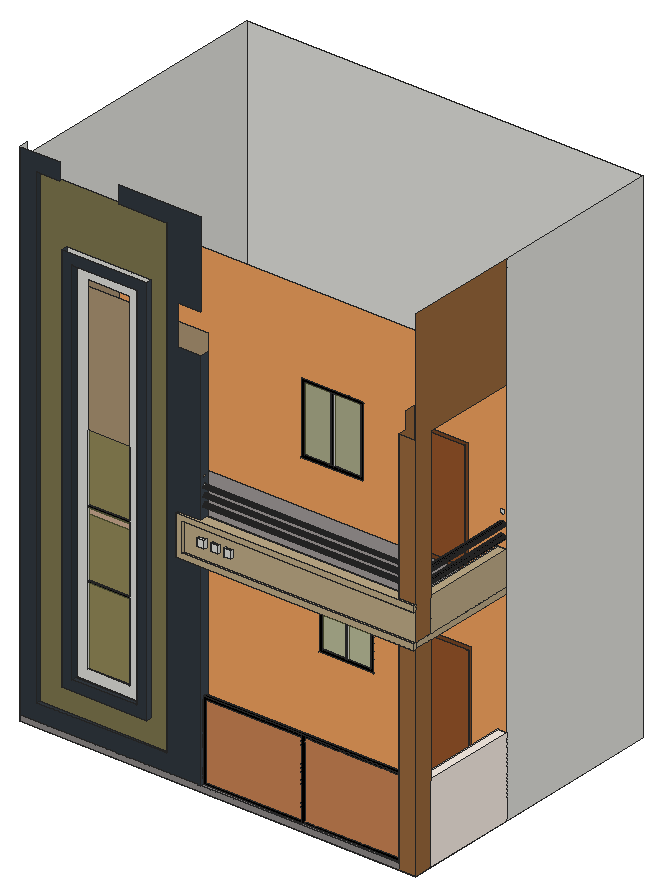
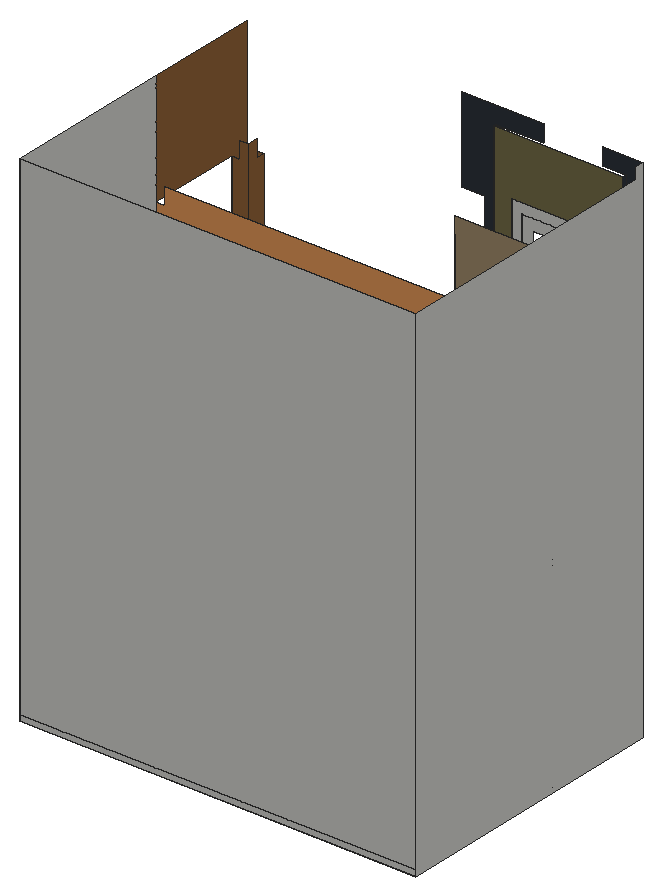
# SketchUp Ruby script. Lengths in inches.
U = 1.inch
M = Sketchup.active_model
def pt(a) = Geom::Point3d.new(a.map { |v| v * U })
def face(e, loops, mat)
  f = e.add_face(loops[0].map { |a| pt(a) })
  loops[1..].each { |l| e.add_face(l.map { |a| pt(a) }).erase! }
  f.material = f.back_material = mat if mat
  f
end
# faces: each face lists its corners as indices into pts; further lists are holes
def faces(e, pts, list, mat = nil) = list.each { |f| face(e, (f[0].is_a?(Array) ? f : [f]).map { |l| l.map { |i| pts[i] } }, mat) }
# xy, xz, yz: faces in a plane at the given z, y or x. An outline is a flat list of corners, or four numbers for a rectangle; further outlines are holes
def ring(l) = l.size == 4 ? [[l[0], l[1]], [l[2], l[1]], [l[2], l[3]], [l[0], l[3]]] : l.each_slice(2).to_a
def flat(e, list, mat, &to3) = list.each { |f| face(e, (f[0].is_a?(Array) ? f : [f]).map { |l| ring(l).map { |u, v| to3.(u, v) } }, mat) }
def xy(e, z, list, mat = nil) = flat(e, list, mat) { |x, y| [x, y, z] }
def xz(e, y, list, mat = nil) = flat(e, list, mat) { |x, z| [x, y, z] }
def yz(e, x, list, mat = nil) = flat(e, list, mat) { |y, z| [x, y, z] }
def lines(e, pts, list) = list.each { |a, b| e.add_line(pt(pts[a]), pt(pts[b])) }
# prism: a flat outline (further loops are holes) pulled along v
def prism(e, loops, v, mat = nil)
  f = face(e, loops, mat); d = Geom::Vector3d.new(v.map { |x| x * U })
  f.pushpull(f.normal.samedirection?(d) ? d.length : -d.length)
end
def box(e, o, s, mat = nil) = prism(e, [[o, [o[0] + s[0], o[1], o[2]], [o[0] + s[0], o[1] + s[1], o[2]], [o[0], o[1] + s[1], o[2]]]], [0, 0, s[2]], mat)
def at(x, y, z, deg = 0) = Geom::Transformation.translation(pt([x, y, z])) * Geom::Transformation.rotation(ORIGIN, Z_AXIS, deg.degrees)
def axes(o, x, y, z) = Geom::Transformation.new([*x, 0, *y, 0, *z, 0, *pt(o).to_a, 1])
def part(name) = M.definitions.add(name)
# library, detail: a bought-in or finely detailed component or shape, given as its bounding box
def library(name, o, s) = part(name).tap { |d| box(d.entities, o, s) }
def detail(e, o, s) = box(e.add_group.entities, o, s)
def put(e, d, t, mat = nil) = e.add_instance(d, t).tap { |i| i.material = mat if mat }
def group(e, t, mat = nil) = e.add_group.tap { |g| g.transformation = t; g.material = mat if mat }.entities
root = M.entities
M.materials.add("[0006_Pink]").color = [255, 192, 203]
M.materials.add("[0008_LavenderBlush]").color = [255, 240, 245]
M.materials.add("[0009_Linen]").color = [250, 240, 230]
M.materials.add("[0032_Moccasin]").color = [193, 173, 137]
M.materials.add("[0033_NavajoWhite]").color = [173, 150, 117]
M.materials.add("[0037_SandyBrown]").color = [244, 164, 96]
M.materials.add("[0111_SlateGray]").color = [49, 56, 63]
M.materials.add("[0111_SlateGray]1").color = [61, 70, 79]
M.materials.add("[0137_Black]").color = [0, 0, 0]
M.materials.add("[Beadboard]").color = [204, 133, 84]
M.materials.add("[Stone Marble]").color = [143, 138, 136]
M.materials.add("[Translucent Glass Gray]").color = [124, 128, 62]
M.materials["[Translucent Glass Gray]"].alpha = 0.5
M.materials.add("[Wood Cherry Original]").color = [152, 86, 42]
M.materials.add("[Wood Floor Dark]").color = [127, 119, 78]
M.materials.add("[Wood Floor]").color = [155, 105, 61]
M.materials.add("[Wood Veneer 01]").color = [120, 70, 37]
xy(root,0,[[0,8,840,608]])
xy(root,12,[[383.22,13.71,802.875,21.28],[635.91,248,758.72,249]])
xy(root,12,[[383.22,8,802.875,13.71],[383.22,21.28,802.875,21.28,802.875,48.0625,821.4375,48.0625,821.4375,248,18,248,18,26,383.22,26]],"[Stone Marble]")
xy(root,48,[[36,8,311.22,14]],"[0111_SlateGray]")
xy(root,99.54,[[93.24,2,272.64,14]],"[0111_SlateGray]1")
xy(root,120.81,[[114.5,2,251.38,14]],"[0111_SlateGray]")
xy(root,144.6,[[138.3,14,227.59,16]])
xy(root,168,[[821.4375,48.0625,840,248]],"[0009_Linen]")
xy(root,180,[[383.22,13.71,802.875,21.28]],"[0137_Black]")
xy(root,187.85,[[449.01,248,498.66,250],[503.92,248,552.48,250]])
xy(root,295.92,[[635.91,248,758.72,249]])
xy(root,297.63,[[449.01,248,498.66,250],[503.92,248,552.48,250]])
xy(root,309.83,[[138.3,14,227.59,16]])
xy(root,312.83,[[138.3,14,227.59,16]])
xy(root,432,[[335.22,2,383.22,8],[383.22,2,802.875,8],[802.875,2,840,8],[425.24,89.85,422.17,90.48,419.37,91.88,417.02,93.96,415.3,96.57,414.31,99.54,414.12,102.67,414.75,105.74,416.15,108.54,418.23,110.88,420.84,112.61,423.82,113.6,426.94,113.79,430.01,113.16,432.8125,111.76,435.16,109.68,436.88,107.06,437.875,104.09,438.0625,100.97,437.43,97.9,436.03,95.09,433.95,92.75,431.34,91.03,428.37,90.04],[545.24,89.85,542.17,90.48,539.37,91.88,537.02,93.96,535.3,96.57,534.31,99.54,534.12,102.67,534.75,105.74,536.15,108.54,538.23,110.88,540.84,112.61,543.82,113.6,546.94,113.79,550.01,113.16,552.8125,111.76,555.16,109.68,556.88,107.06,557.875,104.09,558.0625,100.97,557.43,97.9,556.03,95.09,553.95,92.75,551.34,91.03,548.37,90.04],
  [665.24,89.85,662.17,90.48,659.37,91.88,657.02,93.96,655.3,96.57,654.31,99.54,654.12,102.67,654.75,105.74,656.15,108.54,658.23,110.88,660.84,112.61,663.82,113.6,666.94,113.79,670.01,113.16,672.8125,111.76,675.16,109.68,676.88,107.06,677.875,104.09,678.0625,100.97,677.43,97.9,676.03,95.09,673.95,92.75,671.34,91.03,668.37,90.04]])
xy(root,432,[[[383.22,8,383.22,26,18,26,18,248,840,248,840,48.0625,802.875,48.0625,802.875,8],[545.24,89.85,548.37,90.04,551.34,91.03,553.95,92.75,556.03,95.09,557.43,97.9,558.0625,100.97,557.875,104.09,556.88,107.06,555.16,109.68,552.8125,111.76,550.01,113.16,546.94,113.79,543.82,113.6,540.84,112.61,538.23,110.88,536.15,108.54,534.75,105.74,534.12,102.67,534.31,99.54,535.3,96.57,537.02,93.96,539.37,91.88,542.17,90.48],[665.24,89.85,668.37,90.04,671.34,91.03,673.95,92.75,676.03,95.09,677.43,97.9,678.0625,100.97,677.875,104.09,676.88,107.06,675.16,109.68,672.8125,111.76,670.01,113.16,666.94,113.79,663.82,113.6,660.84,112.61,658.23,110.88,656.15,108.54,654.75,105.74,654.12,102.67,654.31,99.54,655.3,96.57,657.02,93.96,659.37,91.88,662.17,90.48],[425.24,89.85,428.37,90.04,431.34,91.03,433.95,92.75,436.03,95.09,437.43,97.9,438.0625,100.97,437.875,104.09,436.88,107.06,435.16,109.68,432.8125,111.76,430.01,113.16,426.94,113.79,423.82,113.6,420.84,112.61,418.23,110.88,416.15,108.54,414.75,105.74,414.12,102.67,414.31,99.54,415.3,96.57,417.02,93.96,419.37,91.88,422.17,90.48]]],"[0006_Pink]")
xy(root,444,[[383.22,8,802.875,26],[802.875,8,840,48.0625],[821.4375,48.0625,840,248]])
xy(root,444,[[346.875,2,840,8]],"[0032_Moccasin]")
xy(root,444,[[18,26,802.875,26,802.875,48.0625,821.4375,48.0625,821.4375,248,18,248]],"[Stone Marble]")
xy(root,451.35,[[643.26,248,751.37,249]])
xy(root,453.83,[[138.3,14,227.59,16]])
xy(root,456.83,[[138.3,14,227.59,16]])
xy(root,468.74,[[379.9375,2,395.375,8],[408.3125,2,423.75,8],[436.625,2,452.0625,8]])
xy(root,484.18,[[379.9375,2,395.375,8],[408.3125,2,423.75,8],[436.625,2,452.0625,8]])
xy(root,504,[[346.875,2,840,8]],"[0032_Moccasin]")
xy(root,516,[[335.22,2,840,2,840,8,802.875,8,802.875,26,383.22,26,383.22,8,335.22,8],[821.4375,48.0625,840,248]],"[0032_Moccasin]")
xy(root,544.79,[[411.23,248,466.96,249],[473.67,248,530.59,249]])
xz(root,2,[[379.9375,468.74,395.375,484.18],[408.3125,468.74,423.75,484.18],[436.625,468.74,452.0625,484.18]])
xz(root,2,[[335.22,432,840,432,840,444,346.875,444,346.875,504,840,504,840,516,335.22,516]],"[0032_Moccasin]")
xz(root,2,[[[93.24,99.54,272.64,930.88],[114.5,120.81,251.38,909.62]]],"[0111_SlateGray]")
xz(root,8,[[379.9375,468.74,395.375,484.18],[408.3125,468.74,423.75,484.18],[436.625,468.74,452.0625,484.18]])
xz(root,8,[[[346.875,444,840,504],[379.9375,468.74,395.375,484.18],[408.3125,468.74,423.75,484.18],[436.625,468.74,452.0625,484.18]]],"[0032_Moccasin]")
xz(root,8,[[0,12,383.22,12,383.22,432,335.22,432,335.22,516,383.22,516,383.22,828,335.22,828,335.22,912,383.22,912,383.22,1092,209.6,1092,209.6,1056,311.22,1056,311.22,48,36,48,36,1056,85.01,1056,85.01,1092,0,1092]],"[0111_SlateGray]")
xz(root,8,[[0,0,802.875,12]],"[Stone Marble]")
xz(root,8,[[802.875,0,840,432],[802.875,516,840,828]],"[Wood Floor]")
xz(root,13.71,[[383.22,12,589.73,12,589.73,17,388.22,17,388.22,175,589.73,175,589.73,180,383.22,180],[589.73,12,598.66,180],[598.66,12,802.875,12,802.875,180,598.66,180,598.66,175,797.875,175,797.875,17,598.66,17]],"[0137_Black]")
xz(root,13.71,[[388.22,17,589.73,175],[598.66,17,797.875,175]],"[Beadboard]")
xz(root,14,[[[93.24,99.54,272.64,930.88],[114.5,120.81,251.38,909.62]],[[114.5,120.81,251.38,909.62],[138.3,144.6,227.59,885.83]]])
xz(root,14,[[138.3,309.83,227.59,312.83],[138.3,453.83,227.59,456.83]],"[0137_Black]")
xz(root,14,[[[36,48,311.22,1056],[93.24,99.54,272.64,930.88]]],"[Wood Floor Dark]")
xz(root,16,[[138.3,144.6,227.59,309.83],[138.3,312.83,227.59,453.83],[138.3,456.83,227.59,597.83]],"[Translucent Glass Gray]")
xz(root,21.28,[[383.22,12,802.875,180]],"[Beadboard]")
xz(root,26,[[18,12,383.22,432],[18,444,18,864,383.22,864,383.22,516,802.875,516,802.875,444]],"[0033_NavajoWhite]")
xz(root,48.0625,[[821.4375,12,840,168],[821.4375,444,840,516]])
xz(root,48.0625,[[802.875,12,802.875,432,840,432,840,168,821.4375,168,821.4375,12],[[802.875,444,802.875,864,821.4375,864,821.4375,828,840,828,840,516,821.4375,516,821.4375,444],[830.72,579.14,832.27,579.35,833.72,579.95,834.96,580.9,835.91,582.14,836.51,583.59,836.72,585.14,836.51,586.7,835.91,588.14,834.96,589.39,833.72,590.34,832.27,590.9375,830.72,591.14,829.17,590.9375,827.72,590.34,826.48,589.39,825.52,588.14,824.92,586.7,824.72,585.14,824.92,583.59,825.52,582.14,826.48,580.9,827.72,579.95,829.17,579.35],[830.72,555.14,832.27,555.35,833.72,555.95,834.96,556.9,835.91,558.14,836.51,559.59,836.72,561.14,836.51,562.7,835.91,564.14,834.96,565.39,833.72,566.34,832.27,566.9375,830.72,567.14,829.17,566.9375,827.72,566.34,826.48,565.39,825.52,564.14,824.92,562.7,824.72,561.14,824.92,559.59,825.52,558.14,826.48,556.9,827.72,555.95,829.17,555.35],[830.72,531.14,832.27,531.35,833.72,531.95,834.96,532.9,835.91,534.14,836.51,535.59,836.72,537.14,836.51,538.7,835.91,540.14,834.96,541.39,833.72,542.34,832.27,542.9375,830.72,543.14,829.17,542.9375,827.72,542.34,826.48,541.39,825.52,540.14,824.92,538.7,824.72,537.14,824.92,535.59,825.52,534.14,826.48,532.9,827.72,531.95,829.17,531.35]]],"[Wood Floor]")
xz(root,248,[[627.625,3.71,767.01,12],[821.4375,12,840,168],[821.4375,444,840,516],[830.72,531.14,829.17,531.35,827.72,531.95,826.48,532.9,825.52,534.14,824.92,535.59,824.72,537.14,824.92,538.7,825.52,540.14,826.48,541.39,827.72,542.34,829.17,542.9375,830.72,543.14,832.27,542.9375,833.72,542.34,834.96,541.39,835.91,540.14,836.51,538.7,836.72,537.14,836.51,535.59,835.91,534.14,834.96,532.9,833.72,531.95,832.27,531.35],[830.72,555.14,829.17,555.35,827.72,555.95,826.48,556.9,825.52,558.14,824.92,559.59,824.72,561.14,824.92,562.7,825.52,564.14,826.48,565.39,827.72,566.34,829.17,566.9375,830.72,567.14,832.27,566.9375,833.72,566.34,834.96,565.39,835.91,564.14,836.51,562.7,836.72,561.14,836.51,559.59,835.91,558.14,834.96,556.9,833.72,555.95,832.27,555.35]])
xz(root,248,[[[18,12,627.625,12,627.625,304.21,767.01,304.21,767.01,12,821.4375,12,821.4375,168,840,168,840,432,18,432],[442.43,181.27,559.06,304.21]],[[18,444,635.91,444,635.91,690.25,758.72,690.25,758.72,444,821.4375,444,821.4375,516,840,516,840,828,821.4375,828,821.4375,864,18,864],[403.88,537.4375,537.95,690.25],[830.72,531.14,829.17,531.35,827.72,531.95,826.48,532.9,825.52,534.14,824.92,535.59,824.72,537.14,824.92,538.7,825.52,540.14,826.48,541.39,827.72,542.34,829.17,542.9375,830.72,543.14,832.27,542.9375,833.72,542.34,834.96,541.39,835.91,540.14,836.51,538.7,836.72,537.14,836.51,535.59,835.91,534.14,834.96,532.9,833.72,531.95,832.27,531.35],[830.72,555.14,829.17,555.35,827.72,555.95,826.48,556.9,825.52,558.14,824.92,559.59,824.72,561.14,824.92,562.7,825.52,564.14,826.48,565.39,827.72,566.34,829.17,566.9375,830.72,567.14,832.27,566.9375,833.72,566.34,834.96,565.39,835.91,564.14,836.51,562.7,836.72,561.14,836.51,559.59,835.91,558.14,834.96,556.9,833.72,555.95,832.27,555.35],[830.72,579.14,829.17,579.35,827.72,579.95,826.48,580.9,825.52,582.14,824.92,583.59,824.72,585.14,824.92,586.7,825.52,588.14,826.48,589.39,827.72,590.34,829.17,590.9375,830.72,591.14,832.27,590.9375,833.72,590.34,834.96,589.39,835.91,588.14,836.51,586.7,836.72,585.14,836.51,583.59,835.91,582.14,834.96,580.9,833.72,579.95,832.27,579.35]]],"[0037_SandyBrown]")
xz(root,248,[[[442.43,181.27,559.06,304.21],[449.01,187.85,552.48,297.63]],[498.66,187.85,503.92,297.63],[[403.88,537.4375,537.95,690.25],[411.23,544.79,530.59,682.9]],[466.96,544.79,473.67,682.9]],"[0137_Black]")
xz(root,248,[[627.625,12,635.91,12,635.91,295.92,758.72,295.92,758.72,12,767.01,12,767.01,304.21,627.625,304.21],[[635.91,444,758.72,690.25],[643.26,451.35,751.37,682.9]]],"[Wood Veneer 01]")
xz(root,249,[[650.67,134.95,652.22,135.16,653.67,135.76,654.91,136.71,655.86,137.95,656.46,139.4,656.67,140.95,656.46,142.5,655.86,143.95,654.91,145.19,653.67,146.15,652.22,146.75,650.67,146.95,649.11,146.75,647.67,146.15,646.42,145.19,645.47,143.95,644.87,142.5,644.67,140.95,644.87,139.4,645.47,137.95,646.42,136.71,647.67,135.76,649.11,135.16],[652.29,577.41,653.86,577.52,655.34,578.04,656.63,578.92,657.65,580.11,658.34,581.52,658.63,583.06,658.51,584.62,658,586.1,657.12,587.39,655.93,588.42,654.52,589.1,652.98,589.39,651.42,589.27,649.94,588.76,648.65,587.88,647.62,586.69,646.94,585.28,646.65,583.74,646.76,582.18,647.28,580.7,648.16,579.41,649.35,578.38,650.76,577.7]],"[0008_LavenderBlush]")
xz(root,249,[[411.23,544.79,466.96,682.9],[473.67,544.79,530.59,682.9]],"[Translucent Glass Gray]")
xz(root,249,[[[635.91,12,758.72,295.92],[650.67,134.95,649.11,135.16,647.67,135.76,646.42,136.71,645.47,137.95,644.87,139.4,644.67,140.95,644.87,142.5,645.47,143.95,646.42,145.19,647.67,146.15,649.11,146.75,650.67,146.95,652.22,146.75,653.67,146.15,654.91,145.19,655.86,143.95,656.46,142.5,656.67,140.95,656.46,139.4,655.86,137.95,654.91,136.71,653.67,135.76,652.22,135.16]],[[643.26,451.35,751.37,682.9],[652.29,577.41,650.76,577.7,649.35,578.38,648.16,579.41,647.28,580.7,646.76,582.18,646.65,583.74,646.94,585.28,647.62,586.69,648.65,587.88,649.94,588.76,651.42,589.27,652.98,589.39,654.52,589.1,655.93,588.42,657.12,587.39,658,586.1,658.51,584.62,658.63,583.06,658.34,581.52,657.65,580.11,656.63,578.92,655.34,578.04,653.86,577.52]]],"[Wood Cherry Original]")
xz(root,250,[[449.01,187.85,498.66,297.63],[503.92,187.85,552.48,297.63]],"[Translucent Glass Gray]")
xz(root,608,[[0,0,840,12],[0,12,840,1068]])
yz(root,0,[[8,0,8,1092,26,1092,26,1068,608,1068,608,0]])
yz(root,18,[[26,12,248,432],[26,444,248,864]],"[0033_NavajoWhite]")
yz(root,36,[[8,48,14,1056]],"[0111_SlateGray]")
yz(root,93.24,[[2,99.54,14,930.88]],"[0111_SlateGray]1")
yz(root,114.5,[[2,120.81,14,909.62]],"[0111_SlateGray]")
yz(root,138.3,[[14,144.6,16,309.83],[14,312.83,16,453.83],[14,456.83,16,597.83]])
yz(root,227.59,[[14,144.6,16,309.83],[14,312.83,16,453.83],[14,456.83,16,597.83]])
yz(root,251.38,[[2,120.81,14,909.62]],"[0111_SlateGray]")
yz(root,272.64,[[2,99.54,14,930.88]],"[0111_SlateGray]1")
yz(root,311.22,[[8,48,14,1056]],"[0111_SlateGray]")
yz(root,335.22,[[2,432,8,516]])
yz(root,346.875,[[2,444,8,504]],"[0032_Moccasin]")
yz(root,379.9375,[[2,468.74,8,484.18]])
yz(root,383.22,[[13.71,12,21.28,180],[17.13,538.37,16.09,538.47,15.11,538.84,14.26,539.45,13.6,540.26,13.17,541.21,13,542.24,13.1,543.28,13.47,544.25,14.08,545.1,14.89,545.76,15.84,546.2,16.87,546.36,17.91,546.26,18.89,545.89,19.74,545.28,20.4,544.48,20.83,543.53,21,542.49,20.9,541.46,20.53,540.48,19.92,539.63,19.11,538.97,18.16,538.54],[17.13,556.37,16.09,556.47,15.11,556.84,14.26,557.45,13.6,558.26,13.17,559.21,13,560.24,13.1,561.28,13.47,562.25,14.08,563.1,14.89,563.76,15.84,564.2,16.87,564.36,17.91,564.26,18.89,563.89,19.74,563.28,20.4,562.48,20.83,561.53,21,560.49,20.9,559.46,20.53,558.48,19.92,557.63,19.11,556.97,18.16,556.54],[17.13,574.37,16.09,574.47,15.11,574.84,14.26,575.45,13.6,576.26,13.17,577.21,13,578.24,13.1,579.28,13.47,580.25,14.08,581.1,14.89,581.76,15.84,582.2,16.87,582.36,17.91,582.26,18.89,581.89,19.74,581.28,20.4,580.48,20.83,579.53,21,578.49,20.9,577.46,20.53,576.48,19.92,575.63,19.11,574.97,18.16,574.54]])
yz(root,383.22,[[8,12,13.71,12,13.71,180,21.28,180,21.28,12,26,12,26,432,8,432],[[8,516,26,828],[17.13,556.37,16.09,556.47,15.11,556.84,14.26,557.45,13.6,558.26,13.17,559.21,13,560.24,13.1,561.28,13.47,562.25,14.08,563.1,14.89,563.76,15.84,564.2,16.87,564.36,17.91,564.26,18.89,563.89,19.74,563.28,20.4,562.48,20.83,561.53,21,560.49,20.9,559.46,20.53,558.48,19.92,557.63,19.11,556.97,18.16,556.54],[17.13,574.37,16.09,574.47,15.11,574.84,14.26,575.45,13.6,576.26,13.17,577.21,13,578.24,13.1,579.28,13.47,580.25,14.08,581.1,14.89,581.76,15.84,582.2,16.87,582.36,17.91,582.26,18.89,581.89,19.74,581.28,20.4,580.48,20.83,579.53,21,578.49,20.9,577.46,20.53,576.48,19.92,575.63,19.11,574.97,18.16,574.54],[17.13,592.37,16.09,592.47,15.11,592.84,14.26,593.45,13.6,594.26,13.17,595.21,13,596.24,13.1,597.28,13.47,598.25,14.08,599.1,14.89,599.76,15.84,600.2,16.87,600.36,17.91,600.26,18.89,599.89,19.74,599.28,20.4,598.48,20.83,597.53,21,596.49,20.9,595.46,20.53,594.48,19.92,593.63,19.11,592.97,18.16,592.54],[17.13,538.37,16.09,538.47,15.11,538.84,14.26,539.45,13.6,540.26,13.17,541.21,13,542.24,13.1,543.28,13.47,544.25,14.08,545.1,14.89,545.76,15.84,546.2,16.87,546.36,17.91,546.26,18.89,545.89,19.74,545.28,20.4,544.48,20.83,543.53,21,542.49,20.9,541.46,20.53,540.48,19.92,539.63,19.11,538.97,18.16,538.54]]],"[0111_SlateGray]1")
yz(root,395.375,[[2,468.74,8,484.18]])
yz(root,408.3125,[[2,468.74,8,484.18]])
yz(root,411.23,[[248,544.79,249,682.9]])
yz(root,423.75,[[2,468.74,8,484.18]])
yz(root,436.625,[[2,468.74,8,484.18]])
yz(root,449.01,[[248,187.85,250,297.63]])
yz(root,452.0625,[[2,468.74,8,484.18]])
yz(root,466.96,[[248,544.79,249,682.9]])
yz(root,473.67,[[248,544.79,249,682.9]])
yz(root,498.66,[[248,187.85,250,297.63]])
yz(root,503.92,[[248,187.85,250,297.63]])
yz(root,530.59,[[248,544.79,249,682.9]])
yz(root,552.48,[[248,187.85,250,297.63]])
yz(root,635.91,[[248,12,249,295.92]])
yz(root,643.26,[[248,451.35,249,682.9]])
yz(root,751.37,[[248,451.35,249,682.9]])
yz(root,758.72,[[248,12,249,295.92]])
yz(root,802.875,[[13.71,12,21.28,180]])
yz(root,802.875,[[8,12,8,432,48.0625,432,48.0625,12,21.28,12,21.28,180,13.71,180,13.71,12],[[26,444,26,516,8,516,8,828,26,828,26,864,48.0625,864,48.0625,444],[17.13,592.37,18.16,592.54,19.11,592.97,19.92,593.63,20.53,594.48,20.9,595.46,21,596.49,20.83,597.53,20.4,598.48,19.74,599.28,18.89,599.89,17.91,600.26,16.87,600.36,15.84,600.2,14.89,599.76,14.08,599.1,13.47,598.25,13.1,597.28,13,596.24,13.17,595.21,13.6,594.26,14.26,593.45,15.11,592.84,16.09,592.47],[17.13,574.37,18.16,574.54,19.11,574.97,19.92,575.63,20.53,576.48,20.9,577.46,21,578.49,20.83,579.53,20.4,580.48,19.74,581.28,18.89,581.89,17.91,582.26,16.87,582.36,15.84,582.2,14.89,581.76,14.08,581.1,13.47,580.25,13.1,579.28,13,578.24,13.17,577.21,13.6,576.26,14.26,575.45,15.11,574.84,16.09,574.47],[17.13,556.37,18.16,556.54,19.11,556.97,19.92,557.63,20.53,558.48,20.9,559.46,21,560.49,20.83,561.53,20.4,562.48,19.74,563.28,18.89,563.89,17.91,564.26,16.87,564.36,15.84,564.2,14.89,563.76,14.08,563.1,13.47,562.25,13.1,561.28,13,560.24,13.17,559.21,13.6,558.26,14.26,557.45,15.11,556.84,16.09,556.47],[17.13,538.37,18.16,538.54,19.11,538.97,19.92,539.63,20.53,540.48,20.9,541.46,21,542.49,20.83,543.53,20.4,544.48,19.74,545.28,18.89,545.89,17.91,546.26,16.87,546.36,15.84,546.2,14.89,545.76,14.08,545.1,13.47,544.25,13.1,543.28,13,542.24,13.17,541.21,13.6,540.26,14.26,539.45,15.11,538.84,16.09,538.47]]],"[Wood Floor]")
yz(root,821.4375,[[48.0625,444,248,516]])
yz(root,821.4375,[[48.0625,12,248,168]],"[0009_Linen]")
yz(root,840,[[248,0,608,1068]])
yz(root,840,[[48.0625,0,248,168]],"[0009_Linen]")
yz(root,840,[[2,432,8,444],[8,432,248,444],[48.0625,444,248,516],[2,504,8,516]],"[0032_Moccasin]")
yz(root,840,[[8,0,48.0625,432],[8,444,48.0625,444,48.0625,828,248,828,248,1068,8,1068]],"[Wood Floor]")
p = [[829.17,248,531.35],[830.72,248,531.14],[830.72,48.0625,531.14],[829.17,48.0625,531.35],[832.27,248,531.35],[832.27,48.0625,531.35],
  [827.72,248,531.95],[827.72,48.0625,531.95],[833.72,248,531.95],[833.72,48.0625,531.95],[826.48,248,532.9],[826.48,48.0625,532.9],
  [834.96,248,532.9],[834.96,48.0625,532.9],[825.52,248,534.14],[825.52,48.0625,534.14],[835.91,248,534.14],[835.91,48.0625,534.14],
  [824.92,248,535.59],[824.92,48.0625,535.59],[836.51,248,535.59],[836.51,48.0625,535.59],[824.72,248,537.14],[824.72,48.0625,537.14],
  [836.72,248,537.14],[836.72,48.0625,537.14],[824.92,248,538.7],[824.92,48.0625,538.7],[836.51,248,538.7],[836.51,48.0625,538.7],
  [383.22,16.09,538.47],[383.22,17.13,538.37],[802.875,17.13,538.37],[802.875,16.09,538.47],[383.22,18.16,538.54],[802.875,18.16,538.54],
  [383.22,15.11,538.84],[802.875,15.11,538.84],[383.22,19.11,538.97],[802.875,19.11,538.97],[825.52,248,540.14],[825.52,48.0625,540.14],
  [835.91,248,540.14],[835.91,48.0625,540.14],[383.22,14.26,539.45],[802.875,14.26,539.45],[383.22,19.92,539.63],[802.875,19.92,539.63],
  [383.22,13.6,540.26],[802.875,13.6,540.26],[383.22,20.53,540.48],[802.875,20.53,540.48],[826.48,248,541.39],[826.48,48.0625,541.39],
  [834.96,248,541.39],[834.96,48.0625,541.39],[383.22,13.17,541.21],[802.875,13.17,541.21],[383.22,20.9,541.46],[802.875,20.9,541.46],
  [383.22,13,542.24],[802.875,13,542.24],[827.72,248,542.34],[827.72,48.0625,542.34],[833.72,248,542.34],[833.72,48.0625,542.34],
  [383.22,21,542.49],[802.875,21,542.49],[383.22,13.1,543.28],[802.875,13.1,543.28],[829.17,248,542.9375],[829.17,48.0625,542.9375],
  [832.27,248,542.9375],[832.27,48.0625,542.9375],[383.22,20.83,543.53],[802.875,20.83,543.53],[830.72,248,543.14],[830.72,48.0625,543.14],
  [383.22,13.47,544.25],[802.875,13.47,544.25],[383.22,20.4,544.48],[802.875,20.4,544.48],[383.22,14.08,545.1],[802.875,14.08,545.1],
  [383.22,19.74,545.28],[802.875,19.74,545.28],[383.22,14.89,545.76],[802.875,14.89,545.76],[383.22,18.89,545.89],[802.875,18.89,545.89],
  [383.22,15.84,546.2],[802.875,15.84,546.2],[383.22,17.91,546.26],[802.875,17.91,546.26],[383.22,16.87,546.36],[802.875,16.87,546.36],
  [829.17,248,555.35],[830.72,248,555.14],[830.72,48.0625,555.14],[829.17,48.0625,555.35],[832.27,248,555.35],[832.27,48.0625,555.35],
  [827.72,248,555.95],[827.72,48.0625,555.95],[833.72,248,555.95],[833.72,48.0625,555.95],[826.48,248,556.9],[826.48,48.0625,556.9],
  [834.96,248,556.9],[834.96,48.0625,556.9],[383.22,16.09,556.47],[383.22,17.13,556.37],[802.875,17.13,556.37],[802.875,16.09,556.47],
  [383.22,18.16,556.54],[802.875,18.16,556.54],[383.22,15.11,556.84],[802.875,15.11,556.84],[383.22,19.11,556.97],[802.875,19.11,556.97],
  [383.22,14.26,557.45],[802.875,14.26,557.45],[825.52,248,558.14],[825.52,48.0625,558.14],[835.91,248,558.14],[835.91,48.0625,558.14],
  [383.22,19.92,557.63],[802.875,19.92,557.63],[383.22,13.6,558.26],[802.875,13.6,558.26],[383.22,20.53,558.48],[802.875,20.53,558.48],
  [824.92,248,559.59],[824.92,48.0625,559.59],[836.51,248,559.59],[836.51,48.0625,559.59],[383.22,13.17,559.21],[802.875,13.17,559.21],
  [383.22,20.9,559.46],[802.875,20.9,559.46],[383.22,13,560.24],[802.875,13,560.24],[383.22,21,560.49],[802.875,21,560.49],
  [824.72,248,561.14],[824.72,48.0625,561.14],[836.72,248,561.14],[836.72,48.0625,561.14],[383.22,13.1,561.28],[802.875,13.1,561.28],
  [383.22,20.83,561.53],[802.875,20.83,561.53],[824.92,248,562.7],[824.92,48.0625,562.7],[836.51,248,562.7],[836.51,48.0625,562.7],
  [383.22,13.47,562.25],[802.875,13.47,562.25],[383.22,20.4,562.48],[802.875,20.4,562.48],[383.22,14.08,563.1],[802.875,14.08,563.1],
  [383.22,19.74,563.28],[802.875,19.74,563.28],[825.52,248,564.14],[825.52,48.0625,564.14],[835.91,248,564.14],[835.91,48.0625,564.14],
  [383.22,14.89,563.76],[802.875,14.89,563.76],[383.22,18.89,563.89],[802.875,18.89,563.89],[383.22,15.84,564.2],[802.875,15.84,564.2],
  [383.22,17.91,564.26],[802.875,17.91,564.26],[826.48,248,565.39],[826.48,48.0625,565.39],[834.96,248,565.39],[834.96,48.0625,565.39],
  [383.22,16.87,564.36],[802.875,16.87,564.36],[827.72,248,566.34],[827.72,48.0625,566.34],[833.72,248,566.34],[833.72,48.0625,566.34],
  [829.17,248,566.9375],[829.17,48.0625,566.9375],[832.27,248,566.9375],[832.27,48.0625,566.9375],[830.72,248,567.14],[830.72,48.0625,567.14],
  [383.22,16.09,574.47],[383.22,17.13,574.37],[802.875,17.13,574.37],[802.875,16.09,574.47],[383.22,18.16,574.54],[802.875,18.16,574.54],
  [383.22,15.11,574.84],[802.875,15.11,574.84],[383.22,19.11,574.97],[802.875,19.11,574.97],[383.22,14.26,575.45],[802.875,14.26,575.45],
  [383.22,19.92,575.63],[802.875,19.92,575.63],[383.22,13.6,576.26],[802.875,13.6,576.26],[383.22,20.53,576.48],[802.875,20.53,576.48],
  [383.22,13.17,577.21],[802.875,13.17,577.21],[383.22,20.9,577.46],[802.875,20.9,577.46],[383.22,13,578.24],[802.875,13,578.24],
  [383.22,21,578.49],[802.875,21,578.49],[383.22,13.1,579.28],[802.875,13.1,579.28],[383.22,20.83,579.53],[802.875,20.83,579.53],
  [18,248,444],[0,248,444],[18,248,12],[0,248,12],[18,248,432],[0,248,432],
  [383.22,17,542.37],[802.875,17,542.37],[383.22,17,560.37],[802.875,17,560.37],[383.22,17,578.37],[802.875,17,578.37],
  [830.72,248,537.14],[830.72,48.0625,537.14],[830.72,248,561.14],[830.72,48.0625,561.14]]
faces(root,p,[[0,1,2,3],[1,4,5,2],[6,0,3,7],[4,8,9,5],[10,6,7,11],[8,12,13,9],[14,10,11,15],[12,16,17,13],
  [18,14,15,19],[16,20,21,17],[22,18,19,23],[20,24,25,21],[26,22,23,27],[24,28,29,25],[30,31,32,33],[31,34,35,32],
  [36,30,33,37],[34,38,39,35],[40,26,27,41],[28,42,43,29],[44,36,37,45],[38,46,47,39],[48,44,45,49],[46,50,51,47],
  [52,40,41,53],[42,54,55,43],[56,48,49,57],[50,58,59,51],[60,56,57,61],[62,52,53,63],[54,64,65,55],[58,66,67,59],
  [68,60,61,69],[70,62,63,71],[64,72,73,65],[66,74,75,67],[76,70,71,77],[72,76,77,73],[78,68,69,79],[74,80,81,75],
  [82,78,79,83],[80,84,85,81],[86,82,83,87],[84,88,89,85],[90,86,87,91],[88,92,93,89],[94,90,91,95],[92,94,95,93],
  [96,97,98,99],[97,100,101,98],[102,96,99,103],[100,104,105,101],[106,102,103,107],[104,108,109,105],[110,111,112,113],[111,114,115,112],
  [116,110,113,117],[114,118,119,115],[120,116,117,121],[122,106,107,123],[108,124,125,109],[118,126,127,119],[128,120,121,129],[126,130,131,127],
  [132,122,123,133],[124,134,135,125],[136,128,129,137],[130,138,139,131],[140,136,137,141],[138,142,143,139],[144,132,133,145],[134,146,147,135],
  [148,140,141,149],[142,150,151,143],[152,144,145,153],[146,154,155,147],[156,148,149,157],[150,158,159,151],[160,156,157,161],[158,162,163,159],
  [164,152,153,165],[154,166,167,155],[168,160,161,169],[162,170,171,163],[172,168,169,173],[170,174,175,171],[176,164,165,177],[166,178,179,167],
  [180,172,173,181],[174,180,181,175],[182,176,177,183],[178,184,185,179],[186,182,183,187],[184,188,189,185],[190,186,187,191],[188,190,191,189],
  [192,193,194,195],[193,196,197,194],[198,192,195,199],[196,200,201,197],[202,198,199,203],[200,204,205,201],[206,202,203,207],[204,208,209,205],
  [210,206,207,211],[208,212,213,209],[214,210,211,215],[212,216,217,213],[218,214,215,219],[216,220,221,217]],"[0137_Black]")
lines(root,p,[[222,223],[224,225],[226,227],[228,229],[230,231],[232,233],[234,235],[236,237]])
